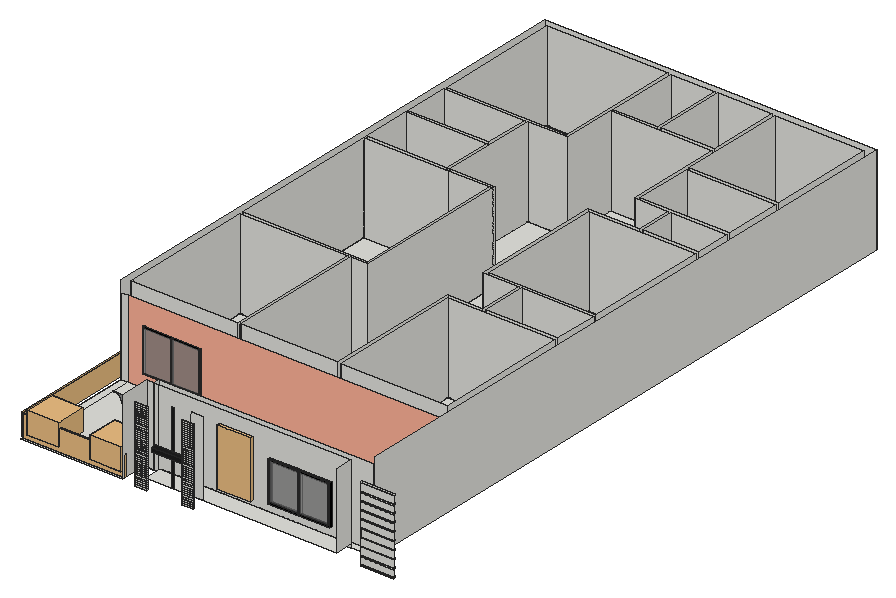
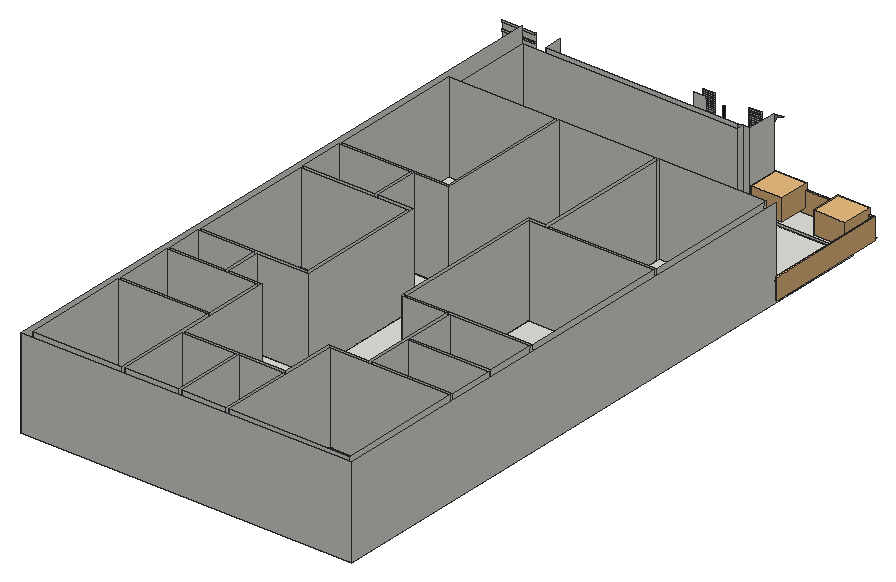
# SketchUp Ruby script. Lengths in inches.
U = 1.inch
M = Sketchup.active_model
def pt(a) = Geom::Point3d.new(a.map { |v| v * U })
def face(e, loops, mat)
  f = e.add_face(loops[0].map { |a| pt(a) })
  loops[1..].each { |l| e.add_face(l.map { |a| pt(a) }).erase! }
  f.material = f.back_material = mat if mat
  f
end
# faces: each face lists its corners as indices into pts; further lists are holes
def faces(e, pts, list, mat = nil) = list.each { |f| face(e, (f[0].is_a?(Array) ? f : [f]).map { |l| l.map { |i| pts[i] } }, mat) }
# xy, xz, yz: faces in a plane at the given z, y or x. An outline is a flat list of corners, or four numbers for a rectangle; further outlines are holes
def ring(l) = l.size == 4 ? [[l[0], l[1]], [l[2], l[1]], [l[2], l[3]], [l[0], l[3]]] : l.each_slice(2).to_a
def flat(e, list, mat, &to3) = list.each { |f| face(e, (f[0].is_a?(Array) ? f : [f]).map { |l| ring(l).map { |u, v| to3.(u, v) } }, mat) }
def xy(e, z, list, mat = nil) = flat(e, list, mat) { |x, y| [x, y, z] }
def xz(e, y, list, mat = nil) = flat(e, list, mat) { |x, z| [x, y, z] }
def yz(e, x, list, mat = nil) = flat(e, list, mat) { |y, z| [x, y, z] }
def lines(e, pts, list) = list.each { |a, b| e.add_line(pt(pts[a]), pt(pts[b])) }
# prism: a flat outline (further loops are holes) pulled along v
def prism(e, loops, v, mat = nil)
  f = face(e, loops, mat); d = Geom::Vector3d.new(v.map { |x| x * U })
  f.pushpull(f.normal.samedirection?(d) ? d.length : -d.length)
end
def box(e, o, s, mat = nil) = prism(e, [[o, [o[0] + s[0], o[1], o[2]], [o[0] + s[0], o[1] + s[1], o[2]], [o[0], o[1] + s[1], o[2]]]], [0, 0, s[2]], mat)
def at(x, y, z, deg = 0) = Geom::Transformation.translation(pt([x, y, z])) * Geom::Transformation.rotation(ORIGIN, Z_AXIS, deg.degrees)
def axes(o, x, y, z) = Geom::Transformation.new([*x, 0, *y, 0, *z, 0, *pt(o).to_a, 1])
def part(name) = M.definitions.add(name)
# library, detail: a bought-in or finely detailed component or shape, given as its bounding box
def library(name, o, s) = part(name).tap { |d| box(d.entities, o, s) }
def detail(e, o, s) = box(e.add_group.entities, o, s)
def put(e, d, t, mat = nil) = e.add_instance(d, t).tap { |i| i.material = mat if mat }
def group(e, t, mat = nil) = e.add_group.tap { |g| g.transformation = t; g.material = mat if mat }.entities
root = M.entities
M.materials.add("[Color B02]").color = [255, 178, 153]
M.materials.add("[Color M04]").color = [142, 142, 142]
M.materials.add("[Color M08]").color = [30, 30, 30]
M.materials.add("[Color_008]").color = [30, 30, 30]
M.materials.add("[Color_009]").color = [0, 0, 0]
M.materials.add("[Translucent_Glass_Gray]").color = [128, 128, 128]
M.materials["[Translucent_Glass_Gray]"].alpha = 0.5
c1 = part("Group\#6")
box(c1.entities,[0,-1.25,0],[15.54,1.25,1.96])
c2 = part("Group\#7")
box(c2.entities,[0,-1.25,0],[16.29,1.25,1.96])
c3 = library("Glass Railings(black Handrails)",[-57.04,-132.55,0],[169.29,2.52,28.17])
c4 = library("plant",[8.5625,309.59,291.73],[41.91,41.15,29.33])
c5 = library("Aluprof_MB-86_Drzwi_panelowe_003_S-0452",[0,0,0],[44.84,5.36,87])
c6 = part("Janela")
xy(c6.entities,0,[[96.33,43.17,179.01,44.35]],"[Color_009]")
xy(c6.entities,1.97,[[98.3,44.15,136.6875,44.35],[138.66,44.15,177.04,44.35]])
xy(c6.entities,1.97,[[98.3,43.17,136.6875,43.46],[138.66,43.17,177.04,43.46]],"[Color_009]")
xy(c6.entities,80.71,[[98.3,43.17,136.6875,43.46],[138.66,43.17,177.04,43.46],[98.3,43.46,136.6875,44.15],[138.66,43.46,177.04,44.15],[98.3,44.15,136.6875,44.35],
  [138.66,44.15,177.04,44.35]])
xy(c6.entities,82.68,[[96.33,43.17,179.01,44.35]],"[Color_008]")
xz(c6.entities,43.17,[[[96.33,0,179.01,82.68],[98.3,1.97,136.6875,80.71],[138.66,1.97,177.04,80.71]]],"[Color_009]")
xz(c6.entities,43.46,[[98.3,1.97,136.6875,80.71],[138.66,1.97,177.04,80.71]],"[Translucent_Glass_Gray]")
xz(c6.entities,44.15,[[98.3,1.97,136.6875,80.71],[138.66,1.97,177.04,80.71]],"[Translucent_Glass_Gray]")
xz(c6.entities,44.35,[[[96.33,0,179.01,82.68],[98.3,1.97,177.04,80.71]],[136.6875,1.97,138.66,80.71]],"[Color_009]")
yz(c6.entities,96.33,[[43.17,0,44.35,82.68]],"[Color_009]")
yz(c6.entities,98.3,[[44.15,1.97,44.35,80.71]])
yz(c6.entities,98.3,[[43.17,1.97,43.46,80.71]],"[Color_009]")
yz(c6.entities,136.6875,[[43.17,1.97,43.46,80.71],[44.15,1.97,44.35,80.71]],"[Color_009]")
yz(c6.entities,138.66,[[43.17,1.97,43.46,80.71],[44.15,1.97,44.35,80.71]])
yz(c6.entities,177.04,[[43.17,1.97,43.46,80.71],[44.15,1.97,44.35,80.71]],"[Color_009]")
yz(c6.entities,179.01,[[43.17,0,44.35,82.68]],"[Color_009]")
xy(root,132,[[[62,205,506,1045],[71,214,497,214,497,518,353,518,353,338,349,338,349,522,397,522,397,582,349,582,349,758,418,758,418,806,373,806,373,936,237,936,237,864,183,864,183,734,179,734,179,800,71,800,71,526,239,526,239,730,243,730,243,522,219,522,219,338,71,338],[71,868,233,1036],[71,342,215,522],[353,586,497,754],[377,892,497,1036],[377,810,497,888],[301,940,373,1036],[71,804,179,864],[237,940,297,1036],[401,522,497,582],[422,758,497,806]]])
xy(root,132.38,[[506,180.5,550.5625,182.5]])
xy(root,132.4375,[[62,205,71,334],[71,205,208.8125,205,208.8125,214,497,214,497,334,71,334],[71,338,215,522],[219,338,349,338,349,522,397,522,397,582,349,582,349,758,418,758,418,806,373,806,373,936,237,936,237,864,183,864,183,734,243,734,243,522,219,522],[353,338,497,518],
  [401,522,497,582],[71,526,239,730],[353,586,497,754],[71,734,179,800],[422,758,497,806],
  [71,804,179,864],[377,810,497,888],[71,868,233,1036],[377,892,497,1036],[237,940,297,1036],
  [301,940,373,1036]])
xy(root,134.38,[[506,180.5,550.5625,182.5]])
xy(root,135.79,[[62,164.8125,199.16,205]])
xy(root,136.625,[[218,180.5,473.75,205]])
xy(root,143.38,[[506,180.5,550.5625,182.5]])
xy(root,145.38,[[506,180.5,550.5625,182.5]])
xy(root,154.38,[[506,180.5,550.5625,182.5]])
xy(root,156.38,[[506,180.5,550.5625,182.5]])
xy(root,165.38,[[506,180.5,550.5625,182.5625]])
xy(root,167.38,[[506,180.5625,550.5625,182.5625]])
xy(root,175.4375,[[231.53,173.5625,278.36,180.5]])
xy(root,176.38,[[506,180.5625,550.5625,182.5]])
xy(root,178.38,[[506,180.5,550.5625,182.5]])
xy(root,180.8125,[[231.53,173.5625,278.36,180.5]],"[Color M08]")
xy(root,187.38,[[506,180.5,550.5625,182.5]])
xy(root,189.38,[[506,180.5,550.5625,182.5]])
xy(root,198.38,[[506,180.5,550.5625,182.5]])
xy(root,200.38,[[506,180.5,550.5625,182.5]])
xy(root,209.38,[[506,180.5,550.5625,182.5]])
xy(root,211.38,[[506,180.5,550.5625,182.5]])
xy(root,220.38,[[506,180.5,550.5625,182.5]])
xy(root,222.38,[[506,180.5,550.5625,182.5]])
xy(root,231.38,[[506,180.5,550.5625,182.5]])
xz(root,164.8125,[[199.16,223.92,199.16,237,186.08,237,187.79,236.89,189.47,236.55,191.09,236,192.62,235.25,194.05,234.3,195.33,233.17,196.46,231.88,197.41,230.46,198.17,228.92,198.72,227.3,199.05,225.625]],"[Color M04]")
xz(root,173.5625,[[231.53,175.4375,278.36,180.8125]],"[Color M08]")
xz(root,180.5,[[506,134.38,550.5625,143.38],[278.36,136.625,278.36,233.875,279.16,233.875,279.16,237,293.91,237,293.91,136.625],[506,145.38,550.5625,154.38],[506,156.38,550.5625,165.38],[506,178.38,550.5625,187.38],
  [506,189.38,550.5625,198.38],[506,200.38,550.5625,209.38],[506,211.38,550.5625,220.38],[506,222.38,550.5625,231.38]])
xz(root,180.5,[[252.06,136.625,254.95,175.4375],[252.06,175.4375,254.95,180.8125],[254.95,175.4375,278.36,180.8125],[252.06,180.8125,254.95,233.875]],"[Color M08]")
xz(root,180.5625,[[506,167.38,550.5625,176.38]])
xz(root,182.5,[[506,132.38,550.5625,134.38],[506,143.38,550.5625,145.38],[506,154.38,550.5625,156.38],[506,176.38,550.5625,178.38],[506,187.38,550.5625,189.38],
  [506,198.38,550.5625,200.38],[506,209.38,550.5625,211.38],[506,220.38,550.5625,222.38],[506,231.38,550.5625,233.38]])
xz(root,182.5625,[[506,165.38,550.5625,167.38]])
xz(root,205,[[62,132,215,132.4375],[215,132,218,132,218,136.625,473.75,136.625,473.75,237,215,237],[218,132,473.75,136.625],[62,132.4375,62,135.79,199.16,135.79,199.16,237,208.8125,237,208.8125,132.4375],[208.8125,132.4375,215,237]])
xz(root,214,[[208.8125,132.4375,497,237]])
xz(root,334,[[62,132.4375,71,237]])
xz(root,334,[[71,132.4375,497,237]],"[Color B02]")
xz(root,338,[[71,132.4375,215,252.4375],[219,132.4375,349,252.4375],[353,132.4375,497,252.4375]])
xz(root,518,[[353,132,497,132.4375],[353,132.4375,497,252.4375]])
xz(root,522,[[71,132,215,132.4375],[219,132,243,132.4375],[349,132,397,132.4375],[401,132,497,132.4375],[71,132.4375,215,252.4375],
  [219,132.4375,243,252.4375],[349,132.4375,397,252.4375],[401,132.4375,497,252.4375]])
xz(root,526,[[71,132,239,132.4375],[71,132.4375,239,252.4375]])
xz(root,582,[[349,132,397,132.4375],[401,132,497,132.4375],[349,132.4375,397,252.4375],[401,132.4375,497,252.4375]])
xz(root,586,[[353,132,497,132.4375],[353,132.4375,497,252.4375]])
xz(root,730,[[239,132,243,252.4375],[71,132.4375,183,252.4375],[183,132.4375,239,252.4375]])
xz(root,734,[[179,132,183,252.4375],[71,132.4375,179,252.4375],[183,132.4375,243,252.4375]])
xz(root,754,[[353,132,497,132.4375],[353,132.4375,497,252.4375]])
xz(root,758,[[349,132,418,132.4375],[422,132,497,132.4375],[349,132.4375,418,252.4375],[422,132.4375,497,252.4375]])
xz(root,800,[[71,132,179,132.4375],[71,132.4375,179,252.4375]])
xz(root,804,[[71,132,179,132.4375],[71,132.4375,179,252.4375]])
xz(root,806,[[373,132,418,132.4375],[422,132,497,132.4375],[373,132.4375,418,252.4375],[422,132.4375,497,252.4375]])
xz(root,810,[[377,132,497,132.4375],[377,132.4375,497,252.4375]])
xz(root,864,[[71,132,179,132.4375],[183,132,237,132.4375],[71,132.4375,179,252.4375],[183,132.4375,237,252.4375]])
xz(root,868,[[71,132,233,132.4375],[71,132.4375,233,252.4375]])
xz(root,888,[[377,132,497,132.4375],[377,132.4375,497,252.4375]])
xz(root,892,[[377,132,497,132.4375],[377,132.4375,497,252.4375]])
xz(root,936,[[237,132,373,132.4375],[237,132.4375,373,252.4375]])
xz(root,940,[[237,132,297,132.4375],[301,132,373,132.4375],[237,132.4375,297,252.4375],[301,132.4375,373,252.4375]])
xz(root,1036,[[71,132,233,132.4375],[237,132,297,132.4375],[301,132,373,132.4375],[377,132,497,132.4375],[71,132.4375,233,252.4375],
  [237,132.4375,297,252.4375],[301,132.4375,373,252.4375],[377,132.4375,497,252.4375]])
xz(root,1045,[[62,132,506,252.4375]])
yz(root,62,[[205,132,205,132.4375,334,132.4375,334,252.4375,1045,252.4375,1045,132]])
yz(root,71,[[342,132,522,132.4375],[526,132,730,132.4375],[730,132,734,252.4375],[734,132,800,132.4375],[804,132,864,132.4375],
  [868,132,1036,132.4375],[338,132.4375,342,252.4375],[342,132.4375,522,252.4375],[526,132.4375,730,252.4375],[734,132.4375,800,252.4375],
  [804,132.4375,864,252.4375],[868,132.4375,1036,252.4375]])
yz(root,179,[[734,132,800,132.4375],[804,132,864,132.4375],[734,132.4375,800,252.4375],[804,132.4375,864,252.4375]])
yz(root,183,[[734,132,864,132.4375],[734,132.4375,864,252.4375]])
yz(root,199.16,[[164.8125,135.79,205,237]])
yz(root,208.8125,[[205,132.4375,214,237]])
yz(root,215,[[342,132,522,132.4375],[338,132.4375,342,252.4375],[342,132.4375,522,252.4375]])
yz(root,219,[[338,132,522,132.4375],[338,132.4375,522,252.4375]])
yz(root,233,[[868,132,1036,132.4375],[868,132.4375,1036,252.4375]])
yz(root,237,[[864,132,936,132.4375],[940,132,1036,132.4375],[864,132.4375,936,252.4375],[940,132.4375,1036,252.4375]])
yz(root,239,[[526,132,730,132.4375],[526,132.4375,730,252.4375]])
yz(root,243,[[522,132,730,132.4375],[522,132.4375,730,252.4375],[730,132.4375,734,252.4375]])
yz(root,297,[[940,132,1036,132.4375],[940,132.4375,1036,252.4375]])
yz(root,301,[[940,132,1036,132.4375],[940,132.4375,1036,252.4375]])
yz(root,349,[[338,132,522,132.4375],[582,132,758,132.4375],[338,132.4375,522,252.4375],[582,132.4375,758,252.4375]])
yz(root,353,[[338,132,518,132.4375],[586,132,754,132.4375],[338,132.4375,518,252.4375],[586,132.4375,754,252.4375]])
yz(root,373,[[806,132,936,132.4375],[940,132,1036,132.4375],[806,132.4375,936,252.4375],[940,132.4375,1036,252.4375]])
yz(root,377,[[810,132,888,132.4375],[892,132,1036,132.4375],[810,132.4375,888,252.4375],[892,132.4375,1036,252.4375]])
yz(root,397,[[522,132,582,132.4375],[522,132.4375,582,252.4375]])
yz(root,401,[[522,132,582,132.4375],[522,132.4375,582,252.4375]])
yz(root,418,[[758,132,806,132.4375],[758,132.4375,806,252.4375]])
yz(root,422,[[758,132,806,132.4375],[758,132.4375,806,252.4375]])
yz(root,473.75,[[180.5,136.625,205,237]])
yz(root,497,[[338,132,518,132.4375],[522,132,582,132.4375],[586,132,754,132.4375],[758,132,806,132.4375],[810,132,888,132.4375],
  [892,132,1036,132.4375],[214,132.4375,334,237],[338,132.4375,518,252.4375],[522,132.4375,582,252.4375],[586,132.4375,754,252.4375],
  [758,132.4375,806,252.4375],[810,132.4375,888,252.4375],[892,132.4375,1036,252.4375]])
yz(root,506,[[205,132,1045,252.4375],[180.5,132.38,182.5,134.38],[180.5,143.38,182.5,145.38],[180.5,154.38,182.5,156.38],[180.5,165.38,182.5625,167.38],
  [180.5,167.38,180.5625,176.38],[180.5,176.38,182.5,178.38],[180.5,187.38,182.5,189.38],[180.5,198.38,182.5,200.38],[180.5,209.38,182.5,211.38],
  [180.5,220.38,182.5,222.38],[180.5,231.38,182.5,233.38]])
p = [[497,214,132.4375],[497,214,132],[71,338,132.4375],[71,338,132],[71,214,132.4375],[71,214,132],
  [505.82,182.32,144.57],[550.38,182.32,144.57]]
lines(root,p,[[0,1],[2,3],[4,5],[6,7]])
put(root,c1,at(278.36,166.5625,132.35))
put(root,c2,at(215.24,166.5625,132.84))
put(root,c1,at(278.36,166.5625,134.91))
put(root,c2,at(215.24,166.5625,135.15))
put(root,c3,axes([108.24,301.04,135.79],[0.81,0,0],[0,1,0],[0,0,1]))
put(root,c3,axes([192.03,280.08,135.83],[0,-0.972,0],[1,0,0],[0,0,1]))
put(root,c1,at(278.36,166.5625,137.28))
put(root,c2,at(215.24,166.5625,137.46))
put(root,c2,at(215.24,166.5625,139.84))
put(root,c1,at(278.36,166.5625,140.16))
put(root,c4,at(60.26,-141.7,-149.9))
put(root,c4,at(144.32,-141.7,-149.9))
put(root,c2,at(215.24,166.5625,142.15))
put(root,c5,axes([297.47,200.49,142.21],[1,0,0],[0,1,0],[0,0,0.89]))
put(root,c1,at(278.36,166.5625,142.85))
put(root,c2,at(215.24,166.5625,144.71))
put(root,c1,at(278.36,166.5625,145.35))
put(root,c2,at(215.24,166.5625,147.27))
put(root,c1,at(278.36,166.5625,147.97))
put(root,c6,axes([269.87,341.4,149.11],[1,0,0],[0,-3.19,0],[0,0,0.6536]))
put(root,c2,at(215.24,166.5625,149.9))
put(root,c1,at(278.36,166.5625,150.41))
put(root,c2,at(215.24,166.5625,152.27))
put(root,c6,axes([3.67,296.875,152.36],[0.94,0,0],[0,0.75,0],[0,0,0.6966]))
put(root,c1,at(278.36,166.5625,152.91))
put(root,c2,at(215.24,166.5625,154.71))
put(root,c1,at(278.36,166.5625,155.47))
put(root,c2,at(215.24,166.5625,157.09))
put(root,c1,at(278.36,166.5625,157.85))
put(root,c2,at(215.24,166.5625,159.52))
put(root,c1,at(278.36,166.5625,160.35))
put(root,c2,at(215.24,166.5625,161.9))
put(root,c1,at(278.36,166.5625,162.85))
put(root,c2,at(215.24,166.5625,164.21))
put(root,c1,at(278.36,166.5625,165.1))
put(root,c2,at(215.24,166.5625,166.46))
put(root,c1,at(278.36,166.5625,167.6))
put(root,c2,at(215.24,166.5625,168.77))
put(root,c1,at(278.36,166.5625,170.1))
put(root,c2,at(215.24,166.5625,171.15))
put(root,c1,at(278.36,166.5625,172.6))
put(root,c2,at(215.24,166.5625,173.46))
put(root,c1,at(278.36,166.5625,175.1))
put(root,c2,at(215.24,166.5625,175.65))
put(root,c1,at(278.36,166.5625,177.53))
put(root,c2,at(215.24,166.5625,177.9))
put(root,c1,at(278.36,166.5625,180.03))
put(root,c2,at(215.24,166.5625,180.21))
put(root,c1,at(278.36,166.5625,182.35))
put(root,c2,at(215.24,166.5625,182.52))
put(root,c2,at(215.24,166.5625,184.71))
put(root,c1,at(278.36,166.5625,184.72))
put(root,c2,at(215.24,166.5625,187.02))
put(root,c1,at(278.36,166.5625,187.03))
put(root,c2,at(215.24,166.5625,189.34))
put(root,c1,at(278.36,166.5625,189.47))
put(root,c2,at(215.24,166.5625,191.65))
put(root,c1,at(278.36,166.5625,191.85))
put(root,c2,at(215.24,166.5625,193.96))
put(root,c1,at(278.36,166.5625,194.16))
put(root,c2,at(215.24,166.5625,196.34))
put(root,c1,at(278.36,166.5625,196.53))
put(root,c2,at(215.24,166.5625,198.71))
put(root,c1,at(278.36,166.5625,198.85))
put(root,c2,at(215.24,166.5625,201.02))
put(root,c1,at(278.36,166.5625,201.16))
put(root,c2,at(215.24,166.5625,203.4))
put(root,c1,at(278.36,166.5625,203.47))
put(root,c1,at(278.36,166.5625,205.85))
put(root,c2,at(215.24,166.5625,205.96))
put(root,c1,at(278.36,166.5625,208.22))
put(root,c2,at(215.24,166.5625,208.27))
put(root,c2,at(215.24,166.5625,210.52))
put(root,c1,at(278.36,166.5625,210.53))
put(root,c1,at(278.36,166.5625,212.91))
put(root,c2,at(215.24,166.5625,213.02))
put(root,c2,at(215.24,166.5625,215.27))
put(root,c1,at(278.36,166.5625,215.28))
put(root,c2,at(215.24,166.5625,217.59))
put(root,c1,at(278.36,166.5625,217.66))
put(root,c2,at(215.24,166.5625,220.02))
put(root,c1,at(278.36,166.5625,220.1))
put(root,c2,at(215.24,166.5625,222.27))
put(root,c1,at(278.36,166.5625,222.47))
put(root,c2,at(215.24,166.5625,224.46))
put(root,c1,at(278.36,166.5625,224.85))
put(root,c2,at(215.24,166.5625,226.71))
put(root,c1,at(278.36,166.5625,227.28))
put(root,c2,at(215.24,166.5625,228.96))
put(root,c1,at(278.36,166.5625,229.6))
put(root,c2,at(215.24,166.5625,231.15))
put(root,c1,at(278.36,166.5625,231.91))
